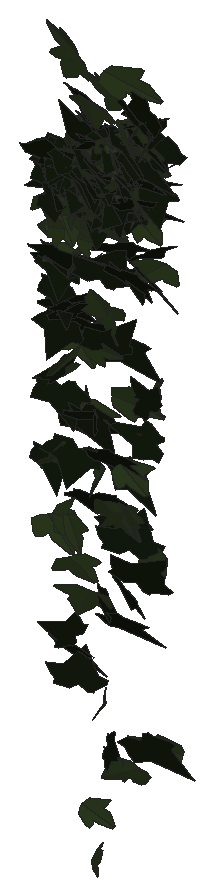
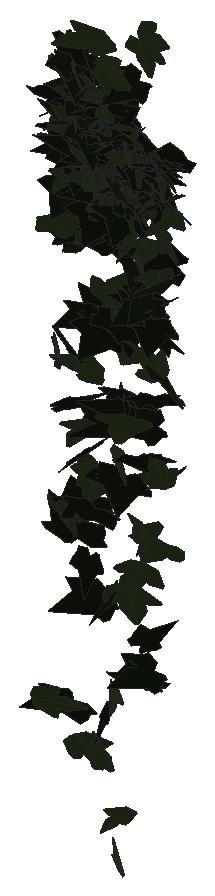
# SketchUp Ruby script. Lengths in millimetres.
U = 1.mm
M = Sketchup.active_model
def pt(a) = Geom::Point3d.new(a.map { |v| v * U })
def face(e, loops, mat)
  f = e.add_face(loops[0].map { |a| pt(a) })
  loops[1..].each { |l| e.add_face(l.map { |a| pt(a) }).erase! }
  f.material = f.back_material = mat if mat
  f
end
# faces: each face lists its corners as indices into pts; further lists are holes
def faces(e, pts, list, mat = nil) = list.each { |f| face(e, (f[0].is_a?(Array) ? f : [f]).map { |l| l.map { |i| pts[i] } }, mat) }
# xy, xz, yz: faces in a plane at the given z, y or x. An outline is a flat list of corners, or four numbers for a rectangle; further outlines are holes
def ring(l) = l.size == 4 ? [[l[0], l[1]], [l[2], l[1]], [l[2], l[3]], [l[0], l[3]]] : l.each_slice(2).to_a
def flat(e, list, mat, &to3) = list.each { |f| face(e, (f[0].is_a?(Array) ? f : [f]).map { |l| ring(l).map { |u, v| to3.(u, v) } }, mat) }
def xy(e, z, list, mat = nil) = flat(e, list, mat) { |x, y| [x, y, z] }
def xz(e, y, list, mat = nil) = flat(e, list, mat) { |x, z| [x, y, z] }
def yz(e, x, list, mat = nil) = flat(e, list, mat) { |y, z| [x, y, z] }
def lines(e, pts, list) = list.each { |a, b| e.add_line(pt(pts[a]), pt(pts[b])) }
# prism: a flat outline (further loops are holes) pulled along v
def prism(e, loops, v, mat = nil)
  f = face(e, loops, mat); d = Geom::Vector3d.new(v.map { |x| x * U })
  f.pushpull(f.normal.samedirection?(d) ? d.length : -d.length)
end
def box(e, o, s, mat = nil) = prism(e, [[o, [o[0] + s[0], o[1], o[2]], [o[0] + s[0], o[1] + s[1], o[2]], [o[0], o[1] + s[1], o[2]]]], [0, 0, s[2]], mat)
def at(x, y, z, deg = 0) = Geom::Transformation.translation(pt([x, y, z])) * Geom::Transformation.rotation(ORIGIN, Z_AXIS, deg.degrees)
def axes(o, x, y, z) = Geom::Transformation.new([*x, 0, *y, 0, *z, 0, *pt(o).to_a, 1])
def part(name) = M.definitions.add(name)
# library, detail: a bought-in or finely detailed component or shape, given as its bounding box
def library(name, o, s) = part(name).tap { |d| box(d.entities, o, s) }
def detail(e, o, s) = box(e.add_group.entities, o, s)
def put(e, d, t, mat = nil) = e.add_instance(d, t).tap { |i| i.material = mat if mat }
def group(e, t, mat = nil) = e.add_group.tap { |g| g.transformation = t; g.material = mat if mat }.entities
root = M.entities
M.materials.add("efeu1").color = [18, 25, 13]
M.materials.add("efeu2").color = [43, 57, 29]
c1 = part("ivyleaf_9")
p = [[39.1,54.8,31.7],[34.5,51.8,30.2],[-5.3,25.2,17.3],[-17.9,28.3,20.9],[-21.6,21.7,17],[-20.2,4.3,5.3],
  [-22.9,-0.3,2.5],[-17.1,-4,-0.6],[-2,-2.1,-1.2],[-0.7,-15.4,-10.1],[16.6,-22.3,-16.7],[21.1,-15.1,-12.5],
  [32.7,-10.7,-11],[46.1,-1.8,-6.6],[30.8,11.2,3.8]]
faces(c1.entities,p,[[0,1,2,3,4,5,6,7,8,9,10,11,12,13,14]],"efeu1")
c2 = part("ivyleaf_10")
p = [[0,12.8,-0.8],[-1.5,51.3,-10.9],[-4.9,51,-11.6],[-13.6,26.5,-7.3],[-13.2,15.9,-4.6],[-21.1,19.3,-7.2],
  [-29.5,16.3,-8.3],[-29.2,8.3,-6.2],[-19.7,-9.8,0.5],[-7.6,-13,4],[1,-12.2,5.8],[-0.4,51.1,-11.1],
  [-1.5,51.1,-10.9],[1,-12.4,5.9],[16.9,-12.4,3.5],[35.1,9.1,-5.1],[35,12.9,-6.1],[20.5,16.4,-4.9],
  [15.8,15,-3.8],[15.3,27.6,-7.1],[12.8,31.3,-7.8]]
faces(c2.entities,p,[[0,1,2,3,4,5,6,7,8,9,10],[11,12,0,13,14,15,16,17,18,19,20]],"efeu2")
put(root,c1,axes([2577.9,1011.3,1295.3],[-0.07296,-0.76074,-0.01951],[0.00206,0.01948,-0.76171],[1.44832,-0.03835,0.0001]))
put(root,c2,axes([2582.9,993.3,1264.9],[-0.57767,-0.53722,-0.50659],[0.62219,0.39334,-0.613],[1.26008,-0.4405,0.07044]))
put(root,c2,axes([2607.5,985.3,1221.1],[0.5573,-0.40858,-0.62654],[-0.71254,0.50243,-0.50262],[1.23242,0.47525,-0.00728]))
put(root,c1,axes([2612.8,995.4,1305.9],[-1.10743,0.49491,0.0287],[-0.04439,0.01687,-0.76388],[-0.94244,-0.58234,0.00226]))
put(root,c1,axes([2577.4,1005.9,1160.2],[1.15557,-0.33842,-0.3488],[-0.31145,0.38321,-0.65667],[0.87094,0.58606,0.22797]))
put(root,c2,axes([2589.3,1007.9,1167.4],[0.60245,0.68252,-0.01434],[-0.04622,-0.00453,-0.75208],[-1.29843,0.31684,0.02012]))
put(root,c1,axes([2584.3,998.3,812],[-0.05249,-0.75428,0.24834],[0.02347,-0.24887,-0.75451],[1.51117,-0.02233,0.02035]))
put(root,c2,axes([2592.6,996.7,807.8],[-0.43136,-0.76206,0.03108],[0.01716,0.02974,0.79505],[-1.45146,0.22683,0.00017]))
put(root,c1,axes([2620,988.2,1348.9],[-0.34918,0.6337,0.41989],[-0.35647,0.38094,-0.65676],[-1.40217,-0.25465,0.06241]))
put(root,c1,axes([2618.1,1003.6,1328.4],[-0.203,0.65874,-0.37637],[-0.21234,-0.38956,-0.6502],[-1.42821,-0.03572,0.15016]))
put(root,c2,axes([2603.2,998.3,718.3],[-0.06202,0.49166,0.71996],[-0.22834,0.71108,-0.49102],[-1.64346,-0.11735,0.04105]))
put(root,c1,axes([2596.6,1005.7,1147.3],[-0.27609,-0.74048,0.20974],[-0.05039,-0.2085,-0.75443],[1.46385,-0.14684,0.01359]))
put(root,c2,axes([2585.4,1001.8,699.1],[1.2814,0.35045,0.38955],[0.66006,0.1774,-0.75903],[-0.74755,0.75736,-0.00246]))
put(root,c1,axes([2605.5,1001.7,1078.5],[1.1318,0.33357,-0.33422],[-0.53049,-0.18585,-0.68146],[-0.72541,0.65636,-0.0231]))
put(root,c2,axes([2596.3,1013.2,1218.3],[0.91905,0.5634,0.16834],[0.14473,0.15616,-0.7408],[-1.10971,0.48697,0.0428]))
put(root,c1,axes([2591.5,1007.1,1312.9],[0.79304,-0.60943,-0.21998],[-0.24212,0.17949,-0.73825],[1.2091,0.43566,-0.00355]))
put(root,c1,axes([2598.2,1006.2,1270.1],[-0.21275,-0.41339,0.63331],[-0.04086,-0.6382,-0.42037],[1.43879,-0.07925,0.08171]))
put(root,c1,axes([2625.3,979.6,988.1],[-0.76591,0.69705,-0.05013],[0.04439,-0.04442,-0.80488],[-1.32932,-0.4031,0.00201]))
put(root,c2,axes([2608.9,995.2,1345],[0.59694,-0.70807,-0.08746],[0.11404,0.12134,-0.76751],[1.35305,0.30216,0.10327]))
put(root,c1,axes([2597.6,976.4,1277.8],[0.73726,-0.26974,-0.66955],[-0.42502,0.67781,-0.40227],[1.30642,0.37274,0.24698]))
put(root,c2,axes([2598.9,1001.6,1319.3],[-0.89993,0.40582,-0.44301],[0.53596,-0.34828,-0.61962],[-1.01002,-0.54639,0.06592]))
put(root,c1,axes([2599,1005.1,1104.4],[-0.1219,-0.7929,0.15389],[0.03776,-0.15587,-0.79485],[1.53675,-0.05907,0.03174]))
put(root,c1,axes([2589.6,1009.4,1284.1],[0.19989,-0.04732,-0.75654],[1.3511,-0.26163,0.11492],[-0.50578,-0.71759,0.00799]))
put(root,c1,axes([2613.1,1003.8,1343.9],[-0.8733,-0.61975,0.07357],[-0.10242,-0.05168,-0.77103],[1.18336,-0.46184,-0.01244]))
put(root,c1,axes([2595.7,1005.7,1309.3],[0.22432,-0.74625,0.12209],[0.10611,-0.11465,-0.75461],[1.43524,0.12511,0.03671]))
put(root,c1,axes([2609.1,1006.1,1332.2],[-1.01201,-0.49871,-0.25576],[0.38536,0.1578,-0.72868],[0.99464,-0.56856,0.0221]))
put(root,c1,axes([2614.2,1001.2,1352.2],[-1.23856,-0.41805,-0.11858],[0.36178,-0.08187,-0.75465],[0.74368,-0.65641,0.16964]))
put(root,c1,axes([2615.9,992.4,1056.8],[-1.36572,-0.02432,-0.39354],[0.74924,0.0014,-0.71793],[0.04187,-0.81842,0.01047]))
put(root,c2,axes([2618.9,1007.1,1328.9],[-0.15354,-0.76041,-0.00077],[-0.00086,0.00083,-0.76468],[1.44721,-0.08067,-0.00054]))
put(root,c2,axes([2637.3,978.5,1544.9],[-0.2304,0.17377,-0.80322],[-0.98305,0.61539,0.21099],[1.21651,0.5302,0.01837]))
put(root,c1,axes([2626.2,1001.3,519.6],[0.04876,0.00766,0.76909],[-1.14825,-0.47707,0.02485],[0.90788,-0.60379,-0.00988]))
put(root,c1,axes([2595.8,1016.8,490],[1.49665,-0.14682,0.00051],[0.00218,0.00332,-0.79997],[0.27943,0.78638,0.00347]))
put(root,c1,axes([2584.4,981.8,1336],[0.33905,-0.06607,0.84503],[1.58131,-0.15713,-0.18745],[0.31898,0.84919,0.03106]))
put(root,c1,axes([2615.3,1006.1,1305.7],[0.9459,-0.25128,-0.5307],[-0.88307,0.25803,-0.55671],[0.68487,0.67976,0.01515]))
put(root,c1,axes([2609,993.3,943.4],[-0.5149,-0.66992,-0.34937],[0.27115,0.3192,-0.72239],[1.41216,-0.30555,0.01132]))
put(root,c1,axes([2584.7,981,1172.6],[1.00022,0.39566,-0.58079],[0.89412,0.34155,0.6578],[0.9947,-0.70488,-0.00727]))
put(root,c2,axes([2615,980.4,980.6],[-0.06776,-0.80114,0.35276],[0.08017,0.35107,0.80156],[-1.66406,0.04953,0.02425]))
put(root,c1,axes([2597.4,1005.3,902.8],[1.31033,-0.34776,0.13065],[0.2235,-0.0573,-0.77133],[0.67078,0.69843,0.00178]))
put(root,c2,axes([2614.7,997.5,1304.8],[-0.52675,0.4977,-0.51593],[0.23792,-0.51106,-0.56006],[-1.34342,-0.28566,0.1031]))
put(root,c1,axes([2621.9,1002.5,1340],[-1.11866,-0.4665,-0.21206],[0.42347,0.05836,-0.74509],[0.87854,-0.62213,0.08912]))
put(root,c2,axes([2624.8,987.7,1301.5],[1.30586,-0.34106,-0.00593],[0.04147,0.05711,-0.76381],[0.64787,0.68378,0.06084]))
put(root,c1,axes([2648.9,994.1,1377.4],[-0.07095,0.17618,0.89989],[-0.46969,0.86548,-0.17967],[-1.6808,-0.24929,0.01222]))
put(root,c2,axes([2630.7,1003.1,1170.8],[0.45166,-0.7524,-0.00097],[-0.00051,0.00093,-0.78894],[1.43197,0.23732,0.00002]))
put(root,c1,axes([2625.8,981.5,1101],[0.60344,0.60748,0.41139],[0.32644,0.37437,-0.68501],[-1.35763,0.36003,0.01815]))
put(root,c1,axes([2629.9,1005.2,838.1],[-0.89248,-0.66083,-0.07989],[0.09878,0.06113,-0.81028],[1.26299,-0.47175,0.00692]))
put(root,c1,axes([2615.5,976.1,1084.7],[0.47481,0.57377,-0.44541],[0.10161,0.45519,0.61627],[1.37867,-0.23115,0.10798]))
put(root,c2,axes([2626.8,1003.1,646.2],[-1.07092,-0.42029,-0.40052],[0.65653,0.2066,-0.70143],[0.88874,-0.65906,0.03554]))
put(root,c2,axes([2645.6,1008.8,1247.4],[-0.50582,0.61137,-0.37942],[-0.2668,0.35273,0.66655],[1.34317,0.3003,-0.01048]))
put(root,c2,axes([2618.3,1000.6,711.7],[1.15154,-0.22591,0.48774],[0.86351,-0.17913,-0.64581],[0.54855,0.75624,-0.00727]))
put(root,c2,axes([2634.5,993.6,1267.9],[0.1058,-0.77018,0.14688],[0.31879,-0.13218,-0.75652],[1.45778,0.0848,0.15478]))
put(root,c2,axes([2641.7,1010.9,1286.9],[-1.02118,-0.52447,0.13192],[0.04554,-0.20867,-0.73229],[1.02825,-0.51162,0.16345]))
put(root,c1,axes([2605.9,988.3,1309.1],[0.72219,-0.21079,0.64558],[1.21997,-0.13309,-0.42023],[0.4269,0.73692,0.10877]))
put(root,c1,axes([2629.7,991.4,1087],[0.66744,0.46919,0.5564],[0.57754,0.46711,-0.58517],[-1.25903,0.463,0.02653]))
put(root,c1,axes([2640.4,996.2,445.2],[-1.24952,0.00947,0.4012],[0.7637,0.00463,0.65654],[0.01078,0.7694,-0.00889]))
put(root,c2,axes([2640.4,981.5,1525.4],[1.37343,-0.32311,-0.20803],[-0.17032,0.28912,-0.7595],[0.71126,0.69315,0.21983]))
put(root,c2,axes([2639.5,989.5,1372.2],[-1.15792,0.48546,-0.09542],[0.05187,-0.11812,-0.77475],[-0.94017,-0.60441,0.07477]))
put(root,c1,axes([2652.4,1001.4,1265.3],[-0.21219,0.75096,-0.08465],[0.05773,-0.08105,-0.75897],[-1.43711,-0.11413,-0.01799]))
put(root,c2,axes([2653.8,1003.4,598],[-1.44389,-0.33026,0.21938],[-0.38234,-0.08816,-0.82743],[0.65056,-0.78481,0.00063]))
put(root,c2,axes([2643.2,1005.5,1203.7],[-0.12249,0.40464,0.6434],[-0.27365,0.62756,-0.40906],[-1.42043,-0.1558,0.02333]))
put(root,c2,axes([2644.8,1004.7,1292.8],[-1.45431,0.04885,-0.02016],[0.03792,-0.00433,-0.76569],[-0.09316,-0.76439,0.00305]))
put(root,c1,axes([2625.6,989.4,1352.7],[0.36231,-0.66032,-0.40509],[0.05776,0.42318,-0.67554],[1.47323,0.1458,0.12611]))
put(root,c2,axes([2643.7,1014.4,1289.9],[1.01861,-0.53839,-0.0603],[-0.07613,0.04526,-0.75914],[1.02825,0.53669,0.00353]))
put(root,c2,axes([2624.7,1013.4,1024.3],[1.26196,0.12344,0.36876],[0.69212,0.06138,-0.67444],[-0.26216,0.75623,-0.00545]))
put(root,c1,axes([2628.2,1010.5,1281.6],[1.07843,-0.46286,-0.20803],[-0.31055,0.12908,-0.73165],[0.91452,0.58966,-0.00313]))
put(root,c2,axes([2640.9,992.7,1341.7],[-0.94207,0.55254,-0.19967],[0.08963,-0.22294,-0.73367],[-1.11455,-0.48496,0.10977]))
put(root,c1,axes([2651,994,1161.1],[0.12188,0.62341,0.42862],[0.09631,0.42566,-0.62667],[-1.43663,0.08142,-0.00565]))
put(root,c2,axes([2653,1008.6,1290.1],[-0.56587,0.64581,-0.29043],[-0.22884,0.26438,0.71096],[1.3281,0.32072,-0.00124]))
put(root,c1,axes([2649.4,1002,1349.6],[0.88321,0.52002,-0.35592],[-0.46541,-0.25876,-0.69691],[-1.10532,0.52447,0.00905]))
put(root,c1,axes([2662.5,1018.9,1299.3],[-0.7861,0.638,-0.06671],[0.06575,-0.0571,-0.76003],[-1.21909,-0.41448,0.00203]))
put(root,c2,axes([2649.3,1001.5,1356.2],[0.09532,-0.78097,-0.0189],[0.00002,0.01894,-0.78257],[1.48677,0.05007,0.00122]))
put(root,c2,axes([2632.2,1019.4,903.4],[1.27135,0.55413,0.27162],[0.38383,0.18227,-0.86785],[-1.11,0.6977,0.011]))
put(root,c1,axes([2643.3,1000.6,1305.8],[-0.70839,-0.64728,0.18796],[0.11716,-0.24647,-0.72685],[1.27743,-0.33634,0.1709]))
put(root,c2,axes([2644.9,1003.1,1351.3],[0.39078,0.72734,0.13381],[-0.16184,0.16117,-0.74558],[-1.39817,0.18463,0.1237]))
put(root,c2,axes([2658.2,990,1357.7],[-1.46555,-0.09821,0.12045],[-0.22217,-0.03643,-0.776],[0.19527,-0.77856,0.02112]))
put(root,c1,axes([2652.3,1010.5,1253.6],[0.83345,0.62601,-0.00664],[-0.08628,0.02363,-0.76229],[-1.18835,0.43733,0.05069]))
put(root,c1,axes([2660.7,1003.9,1064.5],[0.90232,0.4396,-0.42175],[-0.62688,-0.2646,-0.64606],[-0.97534,0.57675,0.02506]))
put(root,c2,axes([2641.1,1007.2,1342.4],[-0.97173,-0.24186,-0.52391],[0.92618,0.19546,-0.56449],[0.59017,-0.70496,0.02323]))
put(root,c2,axes([2666.5,1001.2,1375.1],[1.24954,0.0303,0.42722],[-0.80916,0.14055,0.64341],[-0.09846,-0.7706,0.13415]))
put(root,c2,axes([2662.5,1010.1,1263.3],[-1.14044,-0.4744,0.03321],[-0.02676,-0.03573,-0.76404],[0.90469,-0.59908,0.01927]))
put(root,c2,axes([2650.3,1010.6,224.2],[0.25913,0.58065,0.5233],[0.24511,0.50725,-0.59636],[-1.46733,0.18727,-0.0072]))
put(root,c1,axes([2632.8,1001.5,1290.4],[0.93342,-0.46614,0.3861],[0.61495,-0.21857,-0.67433],[0.97408,0.58467,0.05573]))
put(root,c1,axes([2656.3,1008.2,1290.3],[-0.59683,-0.68107,-0.16899],[0.11577,0.15802,-0.74972],[1.33049,-0.31926,-0.01057]))
put(root,c1,axes([2649.3,996,1316.1],[-0.43545,-0.619,-0.39012],[0.44505,0.32545,-0.65353],[1.31949,-0.31405,0.09168]))
put(root,c1,axes([2648,986.9,1466.5],[1.46838,-0.18345,-0.19129],[-0.34068,0.07354,-0.7925],[0.372,0.79148,0.0293]))
put(root,c1,axes([2674,987.5,898.4],[-0.00805,-0.11342,0.82894],[0.07285,0.82806,0.11349],[-1.59068,0.0385,0.001]))
put(root,c1,axes([2655.2,998.9,1328],[-0.48123,-0.72141,0.01975],[0.21723,-0.06064,-0.75369],[1.35621,-0.24627,0.12773]))
put(root,c2,axes([2654.2,1020.3,135.9],[0.33602,-0.54431,-0.5156],[0.28846,-0.49285,0.5722],[-1.39745,-0.23262,-0.00586]))
put(root,c1,axes([2652.4,1010.3,1297.5],[0.29256,-0.74823,0.02172],[0.01981,-0.02003,-0.76384],[1.4245,0.15395,0.00616]))
put(root,c1,axes([2683.1,997.6,1396.1],[0.28049,-0.27916,0.7209],[-0.54101,0.6629,0.31481],[-1.36822,-0.31935,0.02331]))
put(root,c1,axes([2695.9,1005.3,1303.8],[-1.18688,0.07895,0.4451],[-0.85922,-0.07016,-0.62009],[-0.04381,-0.76296,0.10308]))
put(root,c1,axes([2668.6,995.4,1273.2],[1.03622,0.52606,-0.19868],[-0.26689,-0.14079,-0.75708],[-1.03641,0.56222,-0.00368]))
put(root,c1,axes([2658.1,1000.8,1319.6],[-0.04997,-0.73468,0.27415],[-0.01171,-0.2741,-0.73514],[1.49237,-0.02675,0.00341]))
put(root,c1,axes([2649.3,1001.4,1325.4],[1.27868,-0.36722,0.05072],[0.0849,-0.02414,-0.76566],[0.7004,0.67334,0.00021]))
put(root,c1,axes([2672.9,988.2,782.7],[1.02519,0.54518,-0.24257],[-0.35545,-0.15633,-0.7661],[-1.0786,0.56971,0.02191]))
put(root,c2,axes([2677,981.4,1457.1],[-1.47736,0.1975,0.06938],[-0.12748,0.01811,-0.80098],[-0.37746,-0.77913,-0.00103]))
put(root,c1,axes([2654.5,988.8,919.9],[-0.60453,-0.24491,-0.71185],[1.0644,0.44041,-0.40108],[0.95905,-0.64316,-0.00357]))
put(root,c1,axes([2643.1,987.5,899.3],[0.87128,0.03447,0.66244],[1.26128,0.01109,-0.45857],[-0.05468,0.80516,-0.02205]))
put(root,c2,axes([2671.2,1008.9,1317.7],[0.69733,0.66496,-0.11623],[-0.12438,-0.09668,-0.75915],[-1.2787,0.37203,0.01046]))
put(root,c2,axes([2700.4,1000.5,1474.8],[0.12313,0.16542,-0.9116],[-1.14936,0.70055,0.08426],[1.33723,0.58689,0.15636]))
put(root,c2,axes([2688,1002.9,1093.9],[-1.36259,-0.1147,-0.27326],[-0.51449,-0.04006,0.72507],[-0.23115,0.76528,-0.00301]))
put(root,c1,axes([2658.9,991.6,1367],[0.56364,-0.70332,-0.17221],[-0.03826,0.178,-0.76153],[1.37756,0.29271,0.04931]))
put(root,c2,axes([2681.8,995.1,1283.8],[-0.21293,-0.77393,0.12518],[-0.06873,-0.12123,-0.78176],[1.4905,-0.11615,-0.01817]))
put(root,c1,axes([2670.1,982.5,1424.2],[1.26668,-0.11445,-0.45218],[-0.75866,0.26955,-0.65496],[0.46096,0.75814,0.1646]))
put(root,c1,axes([2653.3,999.7,1367],[1.0361,-0.56867,-0.01587],[0.16266,0.10348,-0.77588],[1.07042,0.53471,0.13327]))
put(root,c2,axes([2681.7,1001.4,422.4],[-0.00592,-0.52012,-0.61428],[-0.05462,0.61397,-0.51971],[1.53092,0.0199,-0.02092]))
put(root,c1,axes([2672.2,1007.9,1261.4],[-0.51644,-0.71818,0.01274],[-0.01577,-0.01048,-0.76772],[1.36696,-0.27145,-0.00404]))
put(root,c1,axes([2672.2,1013.7,595.5],[0.85373,-0.41755,-0.51027],[-0.71716,0.34408,-0.61283],[1.02972,0.58583,-0.00375]))
put(root,c2,axes([2680.8,996.1,817.6],[0.49961,-0.78838,0.02196],[0.01821,-0.01996,-0.83093],[1.50091,0.26267,0.00277]))
put(root,c1,axes([2665.1,997.8,1315.5],[0.78267,-0.62924,-0.14894],[-0.18044,0.11593,-0.75154],[1.21736,0.42174,-0.01563]))
put(root,c2,axes([2655.9,993.9,1247],[-0.41317,-0.05124,-0.74696],[1.42489,-0.00786,-0.21705],[0.01281,-0.77782,0.0514]))
put(root,c1,axes([2670.1,1006.1,1357.9],[0.27487,-0.7539,-0.09451],[-0.00242,0.09596,-0.76743],[1.44605,0.14346,0.01668]))
put(root,c2,axes([2708.5,992.5,1073.8],[-0.07776,0.03215,0.85887],[-1.37421,0.46511,-0.05176],[-0.88726,-0.72319,0.00489]))
put(root,c1,axes([2692.9,983.1,1399.2],[0.49575,0.73966,-0.10409],[-0.05244,-0.10064,-0.78415],[-1.42062,0.26183,-0.00738]))
put(root,c1,axes([2672.1,992.8,1390],[1.5138,0.06777,-0.01492],[-0.03431,0.03606,-0.7974],[-0.12753,0.79472,0.03745]))
put(root,c2,axes([2667.4,987.8,1037.6],[-0.48584,0.03443,0.76724],[1.45492,-0.06623,0.25732],[0.14033,0.80587,-0.01163]))
put(root,c2,axes([2696.5,997.4,1300.9],[-0.72308,-0.67566,-0.15848],[0.15593,0.13574,-0.77514],[1.31159,-0.38863,0.00479]))
put(root,c2,axes([2695.9,1005.6,1276.9],[0.19233,0.5459,-0.5384],[-0.30238,-0.51636,-0.55337],[-1.42757,0.18292,0.04468]))
put(root,c1,axes([2685.6,996.8,1352.1],[-0.06598,-0.77501,0.08013],[-0.02179,-0.07969,-0.77574],[1.4827,-0.03566,-0.00783]))
put(root,c1,axes([2686.3,1014.1,1037.8],[1.42348,0.1255,-0.16887],[-0.32292,-0.00897,-0.75817],[-0.23677,0.76672,0.01877]))
put(root,c2,axes([2701,1005.5,1280.3],[-0.15701,-0.7681,-0.05601],[0.01131,0.05569,-0.77252],[1.46569,-0.08271,-0.00004]))
put(root,c2,axes([2686,990.7,1258.3],[-1.15665,-0.1913,-0.45576],[0.82535,0.14021,-0.63713],[0.45138,-0.7466,-0.00287]))
put(root,c1,axes([2690.3,987,1164.1],[-0.98966,-0.0198,0.64991],[1.23231,-0.09172,0.51527],[0.11294,0.82726,0.07268]))
put(root,c2,axes([2694.1,1023.9,304.6],[-0.98294,0.40191,0.41635],[0.63005,-0.25253,0.65441],[0.90334,0.61345,-0.00339]))
put(root,c2,axes([2702.7,998.6,1339.4],[1.39745,-0.18056,-0.13904],[-0.24433,0.05984,-0.75565],[0.35835,0.74491,0.027]))
put(root,c2,axes([2695.2,989.8,1378.3],[1.43906,0.16138,0.06423],[0.0619,0.15025,-0.76043],[-0.32472,0.74382,0.13967]))
put(root,c1,axes([2678.7,1003,1271.9],[1.21996,0.10651,0.41568],[0.79016,0.03491,-0.64918],[-0.2064,0.76319,-0.02832]))
put(root,c2,axes([2709.9,996.3,1377.5],[-0.27716,-0.7749,-0.08204],[0.0143,0.08206,-0.78843],[1.48297,-0.14562,-0.00773]))
put(root,c1,axes([2684.1,994,1332.1],[1.24319,0.16006,0.40835],[0.69665,0.20462,-0.66573],[-0.45987,0.74267,0.09542]))
put(root,c1,axes([2711.4,978.6,367.9],[0.33217,-0.20926,-0.75548],[-1.0084,0.53894,-0.27169],[1.09959,0.55746,-0.02094]))
put(root,c2,axes([2719.8,996.6,1395],[-0.9979,0.42473,0.41549],[-0.64911,0.23859,-0.67431],[-0.92593,-0.625,0.02494]))
put(root,c2,axes([2716.2,1004.3,1289.1],[-1.3774,0.27178,0.07148],[-0.32093,-0.26201,-0.71111],[-0.42786,-0.67841,0.30328]))
put(root,c2,axes([2707.4,1001.7,1386.4],[0.92079,-0.55944,-0.23219],[0.04425,0.3141,-0.70835],[1.15194,0.43511,0.21281]))
put(root,c2,axes([2732,1012,319.8],[-1.02727,-0.24221,0.56706],[-0.98789,-0.22834,-0.59161],[0.6335,-0.74884,-0.00302]))
put(root,c1,axes([2718.2,1000.8,1297.8],[-1.39205,0.00939,-0.24476],[0.45559,-0.1359,-0.72056],[-0.09876,-0.75923,0.12595]))
put(root,c1,axes([2699.2,1003.5,1379.9],[-0.04643,-0.76512,-0.14188],[-0.00478,0.14203,-0.76548],[1.48099,-0.02353,-0.00692]))
put(root,c1,axes([2685.9,998.7,1383.5],[1.33482,-0.35616,0.06992],[0.30216,0.16424,-0.75595],[0.62119,0.68543,0.21747]))
put(root,c1,axes([2710.5,994.6,1222.6],[1.0159,0.55048,-0.02803],[-0.03614,-0.02063,-0.76678],[-1.04842,0.53412,-0.00073]))
put(root,c1,axes([2701.7,984.7,1048.2],[-0.60693,-0.19137,0.72921],[1.37698,0.14487,0.35443],[-0.40332,0.7826,0.11271]))
put(root,c2,axes([2713.2,1021.7,1297.9],[1.05415,0.50607,-0.15458],[-0.20598,-0.1107,-0.75021],[-0.98579,0.56429,-0.00854]))
put(root,c1,axes([2722.7,1004.9,1361.7],[0.30874,0.75869,0.02151],[0.01392,0.02043,-0.77583],[-1.44445,0.16236,-0.00288]))
put(root,c1,axes([2698.3,977.8,867.2],[1.52348,0.12027,0.1186],[0.22397,0.01495,-0.80946],[-0.23061,0.80908,-0.00268]))
put(root,c2,axes([2727.7,976.1,1371.8],[-0.03188,0.15895,-0.81027],[-0.27428,0.79743,0.15942],[1.54738,0.14462,0.01156]))
put(root,c2,axes([2726.5,1000,1406.6],[-1.46357,0.14951,0.08378],[-0.20072,-0.1092,-0.7731],[-0.25711,-0.76581,0.1266]))
put(root,c1,axes([2709.3,993.1,1307.3],[-0.91436,-0.1502,-0.60604],[1.16471,0.03833,-0.49464],[0.23559,-0.77241,0.0933]))
put(root,c2,axes([2724.4,994.2,1337.3],[0.00483,-0.73929,0.2524],[-0.00185,-0.2524,-0.73929],[1.48676,0.00209,-0.00174]))
put(root,c2,axes([2708.8,993.2,769.2],[-1.50784,0.23188,-0.40705],[0.75136,-0.10004,-0.82539],[-0.47997,-0.88508,-0.01335]))
put(root,c1,axes([2726.1,1002.1,631.5],[0.98596,-0.08659,-0.63464],[-1.16416,0.17525,-0.52323],[0.36162,0.80027,0.04592]))
put(root,c1,axes([2702.2,1021.4,732.5],[-0.40692,-0.31415,-0.6767],[1.01108,0.43013,-0.36753],[0.99692,-0.56447,0.09654]))
put(root,c1,axes([2705.4,1005.6,1345.2],[1.61484,0.08014,0.01658],[0.03145,0.00137,-0.85226],[-0.15255,0.84865,-0.00019]))
put(root,c1,axes([2701.3,1005,572.3],[1.50546,0.05079,0.20048],[0.38089,0.01181,-0.79264],[-0.09921,0.81594,-0.00101]))
put(root,c1,axes([2739.5,995.3,1406],[-0.00954,0.6946,-0.36013],[-0.2075,-0.35724,-0.68752],[-1.47456,0.04578,0.09908]))
put(root,c2,axes([2726.3,993.2,765.5],[-0.56088,-0.69889,-0.32573],[0.24304,0.29965,-0.75848],[1.44722,-0.32118,0.00114]))
put(root,c2,axes([2722.4,996.4,1410.8],[-1.1027,0.52515,-0.13268],[0.1687,-0.09973,-0.78184],[-1.01697,-0.58597,0.01416]))
put(root,c1,axes([2729.1,994.5,1408.9],[-1.04614,-0.5717,-0.01213],[0.01965,0.00689,-0.79308],[1.08813,-0.54976,0.00267]))
put(root,c1,axes([2705.5,988,1352.8],[1.21882,-0.44092,-0.00364],[0.0007,0.00695,-0.77749],[0.83918,0.64038,0.00593]))
put(root,c1,axes([2730.9,1003.1,1298.2],[-1.12308,-0.47787,0.17303],[0.07051,-0.30488,-0.71568],[0.96469,-0.53404,0.25375]))
put(root,c1,axes([2713.1,1019,829.7],[0.49815,-0.78826,-0.38897],[-0.24275,0.36749,-0.83057],[1.65522,0.29113,-0.00475]))
put(root,c2,axes([2718.1,981.3,1410.1],[-0.90234,-0.38208,-0.5098],[0.86808,0.24009,-0.60414],[0.84652,-0.65348,0.07611]))
put(root,c1,axes([2709.5,1001.6,1051.3],[-0.30062,-0.19176,-0.79434],[1.02582,0.58364,-0.24807],[1.16893,-0.5615,0.01342]))
put(root,c2,axes([2736,999.7,1379.5],[-0.52438,-0.45465,0.57869],[0.10459,-0.6289,-0.46794],[1.39671,-0.1236,0.2523]))
put(root,c1,axes([2751.1,996.6,1284.3],[-1.00591,0.55938,-0.10568],[0.10342,-0.09397,-0.76918],[-1.07851,-0.53074,0.02481]))
put(root,c1,axes([2727.1,1001.4,1400.1],[-0.31249,-0.75969,0.03043],[-0.01259,-0.0297,-0.77723],[1.44695,-0.16433,-0.00019]))
put(root,c2,axes([2726.5,991.1,1411.3],[0.7582,0.67987,0.10779],[0.10667,0.09209,-0.78799],[-1.30574,0.4023,-0.00178]))
put(root,c1,axes([2746.1,982,1343.1],[0.07148,0.77603,-0.05707],[-0.06314,-0.05548,-0.77634],[-1.47958,0.03986,0.03037]))
put(root,c2,axes([2738.4,1003.2,1302.3],[0.19472,0.76287,-0.12227],[0.04381,0.12027,0.76967],[1.46977,-0.10465,-0.00674]))
put(root,c1,axes([2734.1,998.2,1377.8],[0.94494,-0.37139,-0.5915],[-0.91617,0.34385,-0.61996],[0.96309,0.69149,-0.0094]))
put(root,c1,axes([2721.7,1016.9,1173.9],[-0.06356,-0.68806,0.37792],[0.35304,-0.37447,-0.66538],[1.45174,0.06094,0.17836]))
put(root,c2,axes([2741.4,1019.5,1330.1],[1.05079,-0.53266,-0.05984],[-0.08545,0.03965,-0.76717],[1.01656,0.55393,-0.00263]))
put(root,c2,axes([2735.9,989.7,1434.3],[-0.14363,0.79789,-0.09432],[0.00031,-0.09472,-0.80141],[-1.52912,-0.07496,0.0087]))
put(root,c1,axes([2719.1,1002.9,1392.8],[1.10136,-0.50888,-0.1274],[0.07174,0.22954,-0.74563],[0.99582,0.54628,0.19463]))
put(root,c2,axes([2735.9,987.2,778.6],[-0.97052,0.62916,-0.16703],[0.19889,-0.13031,-0.80986],[-1.22283,-0.52054,0.00085]))
put(root,c2,axes([2732.6,995,1395.6],[-0.51163,0.54765,-0.50996],[0.41221,-0.46173,-0.61003],[-1.36324,-0.34515,0.00693]))
put(root,c1,axes([2740.4,996,711.5],[-1.19595,-0.15266,0.58918],[1.12808,0.03886,0.64224],[-0.26311,0.86052,0.07552]))
put(root,c1,axes([2727.6,993.8,1415.9],[0.39002,-0.76898,0.07599],[-0.00409,-0.07918,-0.7955],[1.47064,0.20372,-0.02236]))
put(root,c1,axes([2718,1006.7,1328.7],[0.57426,-0.02511,0.70963],[1.33241,0.13936,-0.29275],[-0.22583,0.75842,0.07728]))
put(root,c2,axes([2716.7,991.4,1514.4],[0.63042,0.25516,0.83214],[1.22156,0.52977,-0.41793],[-1.11885,0.72217,0.01257]))
put(root,c2,axes([2755.2,991.4,1431.8],[1.09942,-0.36469,-0.40185],[-0.56116,0.2818,-0.67959],[0.86706,0.64481,0.06972]))
put(root,c1,axes([2749.1,1002.4,1309.8],[0.57277,0.71932,-0.04549],[-0.02003,-0.04491,-0.7797],[-1.37159,0.30104,-0.00761]))
put(root,c1,axes([2763.9,1021.8,888.4],[-0.47796,-0.70114,-0.25858],[-0.08906,-0.2575,0.74366],[-1.41947,0.25224,0.04041]))
put(root,c2,axes([2716.9,1005.1,954],[-0.02749,0.00361,0.82843],[1.54845,0.15616,0.0135],[-0.29704,0.81371,-0.00627]))
put(root,c2,axes([2738.2,989.1,846.9],[0.61537,0.65749,0.38819],[0.27335,0.36166,-0.73219],[-1.42722,0.35275,0.02714]))
put(root,c1,axes([2739.2,978,1192.1],[1.51927,0.11855,-0.17916],[-0.34019,-0.01589,-0.80696],[-0.22679,0.81798,0.01029]))
put(root,c1,axes([2753.6,979.1,1356.1],[0.98597,0.49474,-0.30664],[-0.48425,-0.17672,-0.71499],[-0.99634,0.57549,0.04406]))
put(root,c1,axes([2737,999.1,1402.5],[-0.43051,-0.56696,-0.49776],[0.54581,0.41603,-0.6042],[1.32811,-0.35476,0.08696]))
put(root,c2,axes([2749.8,982.2,1330.1],[-0.84182,0.64076,-0.02802],[0.02241,-0.02592,-0.77858],[-1.22045,-0.44245,0.00503]))
put(root,c2,axes([2757.5,993,1409.9],[-1.4809,-0.06881,0.01909],[-0.03689,0.00248,-0.78114],[0.13081,-0.77834,-0.00418]))
put(root,c1,axes([2743.7,986.7,1356.4],[0.54085,-0.53431,-0.57149],[-0.47392,0.51463,-0.60498],[1.41156,0.37751,0.01586]))
put(root,c1,axes([2749.9,978.9,1471.5],[1.21195,-0.06455,-0.52186],[-0.82783,0.3959,-0.57973],[0.56237,0.72188,0.27128]))
put(root,c1,axes([2764.3,987.1,1453.5],[0.4376,0.77216,0.09879],[-0.09299,0.11712,-0.80172],[-1.47864,0.22116,0.07965]))
put(root,c2,axes([2759.4,991.6,1449.7],[0.43848,-0.76851,0.04333],[0.0187,-0.04229,-0.8023],[1.46484,0.23058,-0.00273]))
put(root,c1,axes([2782.2,988,969.4],[-0.11203,0.32372,0.73238],[-0.36528,0.70724,-0.32804],[-1.47953,-0.19913,0.02553]))
put(root,c2,axes([2777.8,1018.2,1197],[1.07993,0.32209,-0.44924],[-0.92747,-0.01239,-0.62442],[-0.49657,0.72363,0.18927]))
put(root,c1,axes([2786.6,979.4,1487],[0.3227,0.00726,-0.81135],[-1.54416,0.00882,-0.16948],[0.01361,0.82883,0.00891]))
put(root,c1,axes([2750.2,1003.5,1379.6],[0.5185,-0.66723,-0.29761],[-0.01532,0.31487,-0.71329],[1.39038,0.25229,0.10313]))
put(root,c1,axes([2797.3,1006.6,1393.8],[-0.25447,0.26172,0.72516],[-1.36467,0.22815,-0.21455],[-0.539,-0.7012,0.20086]))
put(root,c1,axes([2753,998,657.7],[-0.86149,-0.0354,0.74404],[1.23595,-0.44523,0.37389],[0.69442,0.74851,0.25759]))
put(root,c2,axes([2750.3,1002.6,1312],[-0.67716,-0.29774,0.62876],[0.91733,0.40376,0.46395],[-0.95478,0.59909,-0.00019]))
put(root,c2,axes([2776,1009.8,706.7],[1.22077,-0.42974,-0.25223],[-0.36823,0.16409,-0.7716],[0.87393,0.66942,0.02721]))
put(root,c2,axes([2762.5,997.5,1275.3],[0.41521,0.6149,0.42528],[0.1424,0.42283,-0.64975],[-1.41577,0.22287,0.05937]))
put(root,c2,axes([2769.1,983.2,1336.8],[0.01741,0.77426,0.1015],[-0.12599,0.10191,-0.77142],[-1.48082,0.00043,0.06682]))
put(root,c1,axes([2747.5,973.9,1315.9],[1.26554,0.17182,0.45406],[0.81418,0.15667,-0.68578],[-0.43683,0.7898,0.03726]))
put(root,c2,axes([2800.7,1019.3,372.4],[-0.11446,-0.01271,-0.78677],[-1.49155,-0.06974,0.06103],[-0.13419,0.78598,-0.0073]))
put(root,c2,axes([2763.1,1012,1374.5],[-1.07951,0.38595,-0.36474],[0.50711,-0.25479,-0.68396],[-0.87422,-0.62438,0.05364]))
put(root,c1,axes([2751.2,993.3,1431.1],[0.81888,-0.66631,0.10919],[0.16673,-0.07329,-0.79245],[1.27417,0.43781,0.03352]))
put(root,c1,axes([2760.7,989.3,1347.4],[0.15786,0.78143,0.02976],[-0.00578,-0.0296,0.78582],[1.48829,-0.083,-0.00011]))
put(root,c1,axes([2756,980.8,1396.6],[0.77389,-0.57501,-0.43274],[-0.08095,0.47697,-0.67375],[1.36725,0.3537,0.20505]))
put(root,c2,axes([2763.7,1031,974.7],[0.10441,-0.16322,-0.77629],[0.36761,-0.75197,0.17176],[-1.46429,-0.20042,-0.01224]))
put(root,c1,axes([2751.7,1009.3,1184.6],[0.67522,-0.65507,0.41288],[0.41866,-0.35018,-0.74461],[1.41299,0.41679,0.02332]))
put(root,c1,axes([2796.5,992.5,1447.4],[-1.04883,0.57058,-0.09539],[0.10716,-0.07822,-0.79314],[-1.09577,-0.55379,0.01374]))
put(root,c2,axes([2781.1,988.2,1431.2],[0.47135,-0.75954,-0.00202],[0.01205,0.00419,-0.79886],[1.44551,0.24764,0.00732]))
put(root,c1,axes([2779.3,985.6,1236.8],[0.61141,0.65505,0.26755],[0.22896,0.23899,-0.72958],[-1.32707,0.34303,-0.00261]))
put(root,c1,axes([2758.8,1005.5,378.6],[-0.12334,-0.13453,-0.80919],[1.05166,0.59275,-0.1428],[1.15382,-0.55465,0.04366]))
put(root,c1,axes([2775.5,993,1348.4],[-0.667,-0.6043,-0.39576],[0.40986,0.33247,-0.69837],[1.31228,-0.41099,0.01696]))
